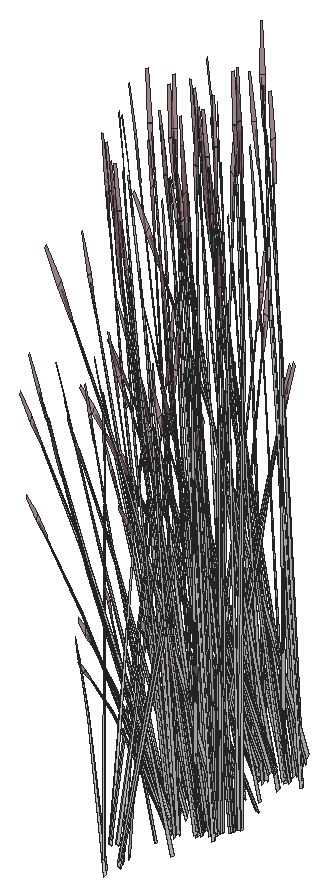
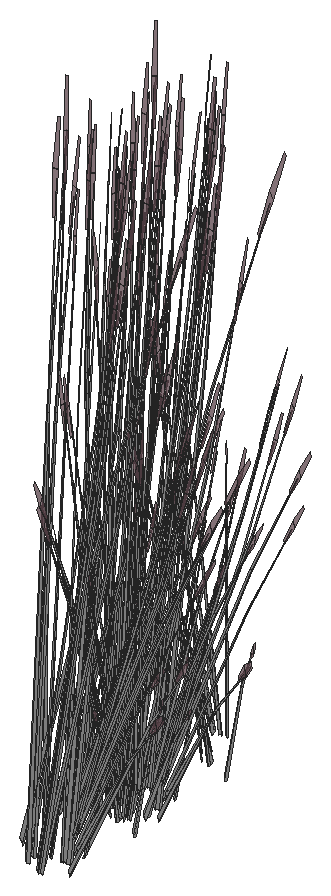
# SketchUp Ruby script. Lengths in inches.
U = 1.inch
M = Sketchup.active_model
def pt(a) = Geom::Point3d.new(a.map { |v| v * U })
def face(e, loops, mat)
  f = e.add_face(loops[0].map { |a| pt(a) })
  loops[1..].each { |l| e.add_face(l.map { |a| pt(a) }).erase! }
  f.material = f.back_material = mat if mat
  f
end
# faces: each face lists its corners as indices into pts; further lists are holes
def faces(e, pts, list, mat = nil) = list.each { |f| face(e, (f[0].is_a?(Array) ? f : [f]).map { |l| l.map { |i| pts[i] } }, mat) }
# xy, xz, yz: faces in a plane at the given z, y or x. An outline is a flat list of corners, or four numbers for a rectangle; further outlines are holes
def ring(l) = l.size == 4 ? [[l[0], l[1]], [l[2], l[1]], [l[2], l[3]], [l[0], l[3]]] : l.each_slice(2).to_a
def flat(e, list, mat, &to3) = list.each { |f| face(e, (f[0].is_a?(Array) ? f : [f]).map { |l| ring(l).map { |u, v| to3.(u, v) } }, mat) }
def xy(e, z, list, mat = nil) = flat(e, list, mat) { |x, y| [x, y, z] }
def xz(e, y, list, mat = nil) = flat(e, list, mat) { |x, z| [x, y, z] }
def yz(e, x, list, mat = nil) = flat(e, list, mat) { |y, z| [x, y, z] }
def lines(e, pts, list) = list.each { |a, b| e.add_line(pt(pts[a]), pt(pts[b])) }
# prism: a flat outline (further loops are holes) pulled along v
def prism(e, loops, v, mat = nil)
  f = face(e, loops, mat); d = Geom::Vector3d.new(v.map { |x| x * U })
  f.pushpull(f.normal.samedirection?(d) ? d.length : -d.length)
end
def box(e, o, s, mat = nil) = prism(e, [[o, [o[0] + s[0], o[1], o[2]], [o[0] + s[0], o[1] + s[1], o[2]], [o[0], o[1] + s[1], o[2]]]], [0, 0, s[2]], mat)
def at(x, y, z, deg = 0) = Geom::Transformation.translation(pt([x, y, z])) * Geom::Transformation.rotation(ORIGIN, Z_AXIS, deg.degrees)
def axes(o, x, y, z) = Geom::Transformation.new([*x, 0, *y, 0, *z, 0, *pt(o).to_a, 1])
def part(name) = M.definitions.add(name)
# library, detail: a bought-in or finely detailed component or shape, given as its bounding box
def library(name, o, s) = part(name).tap { |d| box(d.entities, o, s) }
def detail(e, o, s) = box(e.add_group.entities, o, s)
def put(e, d, t, mat = nil) = e.add_instance(d, t).tap { |i| i.material = mat if mat }
def group(e, t, mat = nil) = e.add_group.tap { |g| g.transformation = t; g.material = mat if mat }.entities
root = M.entities
M.materials.add("LightPink_Translucent").color = [144, 107, 117]
M.materials["LightPink_Translucent"].alpha = 0.75
M.materials.add("[_0053_Ivory_]").color = [200, 200, 200]
c1 = part("blade")
p = [[2.15,0.21,22],[0,0.17,0],[0.09,0.45,0],[2.18,0.31,22],[2.29,0.31,22],[0.38,0.45,0],
  [2.48,0.24,33],[2.49,0.24,33],[2.48,0.22,33]]
faces(c1.entities,p,[[0,1,2,3],[4,5,2,3],[6,3,4,7],[8,0,3,6]])
c2 = part("seeds")
p = [[0.3,-0.1,1.38],[-0.01,-0.03,1.59],[-0.01,-0.03,0.03],[0.14,-0.07,-0.07],[0.29,-0.03,3],[0.15,0.01,3.11]]
faces(c2.entities,p,[[0,1,2,3],[1,0,4,5]],"LightPink_Translucent")
c3 = part("blade with seeds")
put(c3.entities,c1,at(0,0,0))
put(c3.entities,c2,axes([2.4,0.25,30.99],[1.5799,-0.05474,1.17369],[-0.12525,1.92788,0.29478],[-0.07173,-0.02425,1.56792]))
put(root,c3,axes([629.08,314.01,255.53],[0.25192,-0.01424,1.71376],[-0.16712,0.61729,0.13857],[-0.35901,-0.03818,0.73262]),"[_0053_Ivory_]")
put(root,c3,axes([629.08,324.12,255.53],[0.25192,-0.01424,1.71376],[-0.16712,0.61729,0.13857],[-0.35901,-0.03818,0.73262]),"[_0053_Ivory_]")
put(root,c3,axes([629.1875,315.1,255.53],[0.21074,-0.13302,1.71376],[0.17741,0.61464,0.13857],[-0.33083,0.13891,0.73262]),"[_0053_Ivory_]")
put(root,c3,axes([628.53,316.14,254.24],[0.21107,0.05162,1.43002],[0.13604,0.52729,-0.30754],[-0.28671,0.0987,0.61141]),"[_0053_Ivory_]")
put(root,c3,axes([630.4,314.45,255],[0.17264,-0.09097,1.77064],[0.05953,0.63516,0.13857],[-0.37394,0.08428,0.63284]),"[_0053_Ivory_]")
put(root,c3,axes([629.83,313.4375,256.63],[-0.60713,-0.01514,-0.71045],[0.04078,-0.63759,0.08574],[-0.25721,-0.06729,1.00501]),"[_0053_Ivory_]")
put(root,c3,axes([629.83,323.54,256.63],[-0.60713,-0.01514,-0.71045],[0.04078,-0.63759,0.08574],[-0.25721,-0.06729,1.00501]),"[_0053_Ivory_]")
put(root,c3,axes([629.35,313.59,254.24],[0.11858,0.17508,1.43002],[-0.27325,0.4759,-0.30754],[-0.28057,-0.11375,0.61141]),"[_0053_Ivory_]")
put(root,c3,axes([629.35,323.7,254.24],[0.11858,0.17508,1.43002],[-0.27325,0.4759,-0.30754],[-0.28057,-0.11375,0.61141]),"[_0053_Ivory_]")
put(root,c3,axes([628.86,314.54,256.18],[-0.50475,-0.17543,-0.35414],[0.14722,-0.5118,0.4572],[-0.20322,0.04693,0.87481]),"[_0053_Ivory_]")
put(root,c3,axes([628.86,324.65,256.18],[-0.50475,-0.17543,-0.35414],[0.14722,-0.5118,0.4572],[-0.20322,0.04693,0.87481]),"[_0053_Ivory_]")
put(root,c3,axes([629.56,323.125,255.53],[0.2256,0.10835,1.71376],[-0.46687,0.45453,0.13857],[-0.29098,-0.20505,0.73262]),"[_0053_Ivory_]")
put(root,c3,axes([629.21,314.8,256.33],[-0.16454,0.57202,-0.51099],[-0.56413,-0.19607,-0.3958],[-0.22713,0.05245,0.97773]),"[_0053_Ivory_]")
put(root,c3,axes([629.63,313.56,256.33],[-0.44101,0.41656,-0.51099],[-0.38623,-0.44004,-0.3958],[-0.22407,-0.06338,0.97773]),"[_0053_Ivory_]")
put(root,c3,axes([629.63,323.67,256.33],[-0.44101,0.41656,-0.51099],[-0.38623,-0.44004,-0.3958],[-0.22407,-0.06338,0.97773]),"[_0053_Ivory_]")
put(root,c3,axes([628.92,314.76,253.15],[0.0154,0.09911,1.76342],[-0.31051,0.51756,-0.26939],[-0.22056,-0.02609,0.30037]),"[_0053_Ivory_]")
put(root,c3,axes([628.92,324.87,253.15],[0.0154,0.09911,1.76342],[-0.31051,0.51756,-0.26939],[-0.22056,-0.02609,0.30037]),"[_0053_Ivory_]")
put(root,c3,axes([628.09,317.25,254.42],[0.25312,-0.28501,1.1486],[0.09988,0.45119,0.84392],[-0.18292,0.08079,0.25299]),"[_0053_Ivory_]")
put(root,c3,axes([629.47,313.17,256.18],[-0.34557,-0.39372,-0.35414],[0.39459,-0.37271,0.4572],[-0.20048,-0.05671,0.87481]),"[_0053_Ivory_]")
put(root,c3,axes([629.47,323.28,256.18],[-0.34557,-0.39372,-0.35414],[0.39459,-0.37271,0.4572],[-0.20048,-0.05671,0.87481]),"[_0053_Ivory_]")
put(root,c3,axes([629.96,315.51,255.53],[0.1517,-0.19322,1.71376],[0.38303,0.52154,0.13857],[-0.26271,0.23751,0.73262]),"[_0053_Ivory_]")
put(root,c3,axes([629.04,316.02,256.18],[-0.52868,0.08987,-0.35414],[-0.1396,-0.51376,0.4572],[-0.1515,0.13799,0.87481]),"[_0053_Ivory_]")
put(root,c3,axes([628.76,307.15,253.15],[0.08147,0.06283,1.76342],[0.13814,0.58211,-0.26939],[-0.18056,0.12413,0.30037]),"[_0053_Ivory_]")
put(root,c3,axes([628.76,317.54,253.15],[0.08147,0.06283,1.76342],[0.13814,0.58211,-0.26939],[-0.18056,0.12413,0.30037]),"[_0053_Ivory_]")
put(root,c3,axes([628.64,314.12,254.42],[0.38775,-0.045,1.1486],[-0.24596,0.39648,0.84392],[-0.19161,-0.05948,0.25299]),"[_0053_Ivory_]")
put(root,c3,axes([628.64,324.22,254.42],[0.38775,-0.045,1.1486],[-0.24596,0.39648,0.84392],[-0.19161,-0.05948,0.25299]),"[_0053_Ivory_]")
put(root,c3,axes([629.84,305.6,255.53],[0.11309,-0.21615,1.71376],[0.47441,0.44731,0.13857],[-0.21402,0.27879,0.73262]),"[_0053_Ivory_]")
put(root,c3,axes([629.84,315.99,255.53],[0.11309,-0.21615,1.71376],[0.47441,0.44731,0.13857],[-0.21402,0.27879,0.73262]),"[_0053_Ivory_]")
put(root,c3,axes([629.48,316.08,256.33],[0.15602,0.5742,-0.51099],[-0.59087,0.10045,-0.3958],[-0.16933,0.15423,0.97773]),"[_0053_Ivory_]")
put(root,c3,axes([630.95,315.66,253.71],[-0.63179,-0.1031,-0.62353],[0.13332,-0.63596,-0.16365],[-0.18854,-0.07706,1.37633]),"[_0053_Ivory_]")
put(root,c3,axes([630.95,325.77,253.71],[-0.63179,-0.1031,-0.62353],[0.13332,-0.63596,-0.16365],[-0.18854,-0.07706,1.37633]),"[_0053_Ivory_]")
put(root,c3,axes([630.89,322.79,256.63],[-0.51789,-0.30395,-0.71045],[0.36805,-0.53263,0.08574],[-0.18764,-0.18149,1.00501]),"[_0053_Ivory_]")
put(root,c3,axes([630.65,312.7,256.33],[-0.59932,0.14948,-0.51099],[-0.10484,-0.56611,-0.3958],[-0.16097,-0.16223,0.97773]),"[_0053_Ivory_]")
put(root,c3,axes([630.65,322.81,256.33],[-0.59932,0.14948,-0.51099],[-0.10484,-0.56611,-0.3958],[-0.16097,-0.16223,0.97773]),"[_0053_Ivory_]")
put(root,c3,axes([630.125,316.87,253.67],[-0.56842,-0.31443,-0.49651],[0.33976,-0.56381,0],[-0.12946,-0.07161,1.57504]),"[_0053_Ivory_]")
put(root,c3,axes([630.125,326.97,253.67],[-0.56842,-0.31443,-0.49651],[0.33976,-0.56381,0],[-0.12946,-0.07161,1.57504]),"[_0053_Ivory_]")
put(root,c3,axes([629.875,322.29,253.15],[-0.05883,0.08284,1.76342],[-0.59454,0.17861,-0.26939],[-0.14363,-0.16248,0.30037]),"[_0053_Ivory_]")
put(root,c3,axes([630.47,317.25,254.03],[-0.37973,0.63014,0],[-0.6353,-0.35142,-0.51607],[-0.14469,-0.08004,1.63711]),"[_0053_Ivory_]")
put(root,c3,axes([629.78,307.77,254.24],[0.19166,-0.0992,1.43002],[0.4732,0.29912,-0.30754],[-0.14084,0.25882,0.61141]),"[_0053_Ivory_]")
put(root,c3,axes([629.78,318.16,254.24],[0.19166,-0.0992,1.43002],[0.4732,0.29912,-0.30754],[-0.14084,0.25882,0.61141]),"[_0053_Ivory_]")
put(root,c3,axes([629.51,312.5,253.78],[-0.1752,0.51349,-0.03893],[-0.53924,-0.15795,-0.17649],[-0.08187,-0.08399,0.58215]),"[_0053_Ivory_]")
put(root,c3,axes([629.51,322.61,253.78],[-0.1752,0.51349,-0.03893],[-0.53924,-0.15795,-0.17649],[-0.08187,-0.08399,0.58215]),"[_0053_Ivory_]")
put(root,c3,axes([630.3125,321.96,254.24],[-0.03678,0.20572,1.43002],[-0.53767,0.17221,-0.30754],[-0.12568,-0.26589,0.61141]),"[_0053_Ivory_]")
put(root,c3,axes([630.49,322.49,255.53],[0.13883,0.2019,1.71376],[-0.64153,0.16998,0.13857],[-0.14499,-0.31697,0.73262]),"[_0053_Ivory_]")
put(root,c3,axes([631.67,315.76,254.32],[-0.61322,0.4175,-0.29095],[-0.40778,-0.58992,-0.50002],[-0.1513,-0.05991,1.59708]),"[_0053_Ivory_]")
put(root,c3,axes([630.71,322.39,256.18],[-0.0938,-0.50652,-0.35414],[0.53623,-0.13375,0.4572],[-0.14403,-0.14515,0.87481]),"[_0053_Ivory_]")
put(root,c3,axes([629.22,314.85,254.03],[-0.75945,0,0],[0,-0.70283,-0.51607],[0,-0.16007,1.63711]),"[_0053_Ivory_]")
put(root,c3,axes([629.22,324.95,254.03],[-0.75945,0,0],[0,-0.70283,-0.51607],[0,-0.16007,1.63711]),"[_0053_Ivory_]")
put(root,c3,axes([630.28,316.63,253.68],[-0.14267,-0.54795,-0.30978],[0.56663,-0.1556,0.30978],[-0.11423,-0.06319,1.38974]),"[_0053_Ivory_]")
put(root,c3,axes([630.28,326.74,253.68],[-0.14267,-0.54795,-0.30978],[0.56663,-0.1556,0.30978],[-0.11423,-0.06319,1.38974]),"[_0053_Ivory_]")
put(root,c3,axes([629.97,306.8125,256.18],[-0.41095,0.33109,-0.35414],[-0.38901,-0.37805,0.4572],[-0.05919,0.19208,0.87481]),"[_0053_Ivory_]")
put(root,c3,axes([629.97,317.2,256.18],[-0.41095,0.33109,-0.35414],[-0.38901,-0.37805,0.4572],[-0.05919,0.19208,0.87481]),"[_0053_Ivory_]")
put(root,c3,axes([632.08,316.21,253.71],[-0.40909,0.47266,-0.62353],[-0.50819,-0.4286,-0.16365],[-0.16393,0.11791,1.37633]),"[_0053_Ivory_]")
put(root,c3,axes([629.8,314.66,253.98],[-0.56493,0.5287,0.30756],[-0.56528,-0.52313,-0.36492],[-0.01973,-0.15014,1.64885]),"[_0053_Ivory_]")
put(root,c3,axes([629.8,324.77,253.98],[-0.56493,0.5287,0.30756],[-0.56528,-0.52313,-0.36492],[-0.01973,-0.15014,1.64885]),"[_0053_Ivory_]")
put(root,c3,axes([632.13,316.12,254.98],[0.52485,0.25358,1.51261],[-0.51417,0.54629,0.59816],[-0.23031,-0.32378,1.26806]),"[_0053_Ivory_]")
put(root,c3,axes([632.13,326.23,254.98],[0.52485,0.25358,1.51261],[-0.51417,0.54629,0.59816],[-0.23031,-0.32378,1.26806]),"[_0053_Ivory_]")
put(root,c3,axes([630.125,321.63,254.42],[0.31682,0.21887,1.1486],[-0.4614,0.13157,0.84392],[-0.09872,-0.16821,0.25299]),"[_0053_Ivory_]")
put(root,c3,axes([632.36,315.95,254.12],[-0.59306,-0.50614,-0.25192],[0.49904,-0.56836,0.5513],[-0.1597,0.05921,1.68216]),"[_0053_Ivory_]")
put(root,c3,axes([631.28,315.46,253.86],[-0.36485,-0.52782,-0.44739],[0.55265,-0.37168,0.21531],[-0.11807,-0.06531,1.43643]),"[_0053_Ivory_]")
put(root,c3,axes([631.28,325.57,253.86],[-0.36485,-0.52782,-0.44739],[0.55265,-0.37168,0.21531],[-0.11807,-0.06531,1.43643]),"[_0053_Ivory_]")
put(root,c3,axes([630.25,306.46,256.99],[-0.0158,0.58168,-0.7886],[-0.66548,-0.03907,0.09517],[-0.07023,0.24643,1.11556]),"[_0053_Ivory_]")
put(root,c3,axes([630.25,316.85,256.99],[-0.0158,0.58168,-0.7886],[-0.66548,-0.03907,0.09517],[-0.07023,0.24643,1.11556]),"[_0053_Ivory_]")
put(root,c3,axes([630.24,308.1,254.42],[-0.01572,-0.37392,1.1486],[0.39276,0.26669,0.84392],[-0.07724,0.17822,0.25299]),"[_0053_Ivory_]")
put(root,c3,axes([630.24,318.49,254.42],[-0.01572,-0.37392,1.1486],[0.39276,0.26669,0.84392],[-0.07724,0.17822,0.25299]),"[_0053_Ivory_]")
put(root,c3,axes([632.06,315.84,253.86],[-0.65953,0.03882,-0.44739],[-0.05964,-0.64439,0.21531],[-0.11807,0.06531,1.43643]),"[_0053_Ivory_]")
put(root,c3,axes([630.8,316.92,254.13],[0.56842,0.31443,0.49651],[-0.33976,0.56381,0],[-0.12946,-0.07161,1.57504]),"[_0053_Ivory_]")
put(root,c3,axes([630.03,307.28,255.02],[0.01334,-0.32463,1.54345],[0.60018,0.17147,0.21329],[-0.052,0.34598,0.72882]),"[_0053_Ivory_]")
put(root,c3,axes([630.03,317.67,255.02],[0.01334,-0.32463,1.54345],[0.60018,0.17147,0.21329],[-0.052,0.34598,0.72882]),"[_0053_Ivory_]")
put(root,c3,axes([631.33,315.76,254.09],[0.16098,-0.74515,-0.23429],[0.76326,0.12989,0.51271],[-0.13337,-0.1029,1.5644]),"[_0053_Ivory_]")
put(root,c3,axes([631.33,325.87,254.09],[0.16098,-0.74515,-0.23429],[0.76326,0.12989,0.51271],[-0.13337,-0.1029,1.5644]),"[_0053_Ivory_]")
put(root,c3,axes([631.61,315.94,254.27],[-0.11717,0.56122,0.1448],[-0.57245,-0.09742,-0.41347],[-0.10418,-0.05763,1.26744]),"[_0053_Ivory_]")
put(root,c3,axes([632.75,317.5,253.67],[-0.56842,0.31443,-0.49651],[-0.33976,-0.56381,0],[-0.12946,0.07161,1.57504]),"[_0053_Ivory_]")
put(root,c3,axes([629.39,314.37,253.67],[0,-0.62885,-0.49651],[0.67951,0,0],[0,-0.14322,1.57504]),"[_0053_Ivory_]")
put(root,c3,axes([629.39,324.48,253.67],[0,-0.62885,-0.49651],[0.67951,0,0],[0,-0.14322,1.57504]),"[_0053_Ivory_]")
put(root,c3,axes([629.68,314.95,254.13],[0,0.62885,0.49651],[-0.67951,0,0],[0,-0.14322,1.57504]),"[_0053_Ivory_]")
put(root,c3,axes([629.68,325.06,254.13],[0,0.62885,0.49651],[-0.67951,0,0],[0,-0.14322,1.57504]),"[_0053_Ivory_]")
put(root,c3,axes([632.79,317.33,253.85],[-0.37499,-0.63235,-0.05142],[0.6353,-0.35142,0.51607],[-0.15655,0.0602,1.6363]),"[_0053_Ivory_]")
put(root,c3,axes([630.38,306.66,256.66],[0.43478,0.42253,-0.5672],[-0.45929,0.37004,-0.43934],[-0.06615,0.21468,1.08528]),"[_0053_Ivory_]")
put(root,c3,axes([630.38,317.05,256.66],[0.43478,0.42253,-0.5672],[-0.45929,0.37004,-0.43934],[-0.06615,0.21468,1.08528]),"[_0053_Ivory_]")
put(root,c3,axes([632.62,317.25,253.68],[-0.56663,-0.1556,-0.30978],[0.14267,-0.54795,0.30978],[-0.11423,0.06319,1.38974]),"[_0053_Ivory_]")
put(root,c3,axes([631.16,315.1,254.32],[-0.68399,-0.30005,-0.29095],[0.32934,-0.63331,-0.50002],[-0.0215,-0.15549,1.59708]),"[_0053_Ivory_]")
put(root,c3,axes([631.16,325.2,254.32],[-0.68399,-0.30005,-0.29095],[0.32934,-0.63331,-0.50002],[-0.0215,-0.15549,1.59708]),"[_0053_Ivory_]")
put(root,c3,axes([632.94,314.91,254.5],[-0.01659,-0.59209,1.41272],[0.75089,0.15348,0.59816],[-0.1776,0.32398,1.3335]),"[_0053_Ivory_]")
put(root,c3,axes([629.91,307.29,254.48],[0.55175,-0.11136,0.06507],[0.12684,0.44864,-0.86304],[-0.03498,0.22711,0.7736]),"[_0053_Ivory_]")
put(root,c3,axes([629.91,317.68,254.48],[0.55175,-0.11136,0.06507],[0.12684,0.44864,-0.86304],[-0.03498,0.22711,0.7736]),"[_0053_Ivory_]")
put(root,c3,axes([632.52,315.67,254.32],[0.07077,0.71755,-0.29095],[-0.73712,0.04339,-0.50002],[-0.1298,0.09558,1.59708]),"[_0053_Ivory_]")
put(root,c3,axes([630.86,324.57,253.75],[-0.24943,-0.64486,-0.69835],[0.71849,-0.23224,-0.18329],[-0.02757,-0.21836,1.54149]),"[_0053_Ivory_]")
put(root,c3,axes([631.98,322.54,256.33],[-0.59704,-0.15764,-0.51099],[0.20464,-0.54049,-0.3958],[-0.05475,-0.21761,0.97773]),"[_0053_Ivory_]")
put(root,c3,axes([630.88,306.05,255.53],[-0.01487,-0.24136,1.71376],[0.64429,0.16012,0.13857],[-0.03985,0.34396,0.73262]),"[_0053_Ivory_]")
put(root,c3,axes([630.88,316.44,255.53],[-0.01487,-0.24136,1.71376],[0.64429,0.16012,0.13857],[-0.03985,0.34396,0.73262]),"[_0053_Ivory_]")
put(root,c3,axes([629.68,314.38,253.68],[0.42396,-0.39235,-0.30978],[0.42396,0.39235,0.30978],[0,-0.12637,1.38974]),"[_0053_Ivory_]")
put(root,c3,axes([629.68,324.49,253.68],[0.42396,-0.39235,-0.30978],[0.42396,0.39235,0.30978],[0,-0.12637,1.38974]),"[_0053_Ivory_]")
put(root,c3,axes([631.59,311.85,253.78],[-0.4197,0.36076,-0.03893],[-0.38456,-0.39511,-0.17649],[-0.02707,-0.11196,0.58215]),"[_0053_Ivory_]")
put(root,c3,axes([631.59,321.95,253.78],[-0.4197,0.36076,-0.03893],[-0.38456,-0.39511,-0.17649],[-0.02707,-0.11196,0.58215]),"[_0053_Ivory_]")
put(root,c3,axes([631.42,315.4,254.01],[0.76764,0.13249,0.45755],[-0.15622,0.74829,0.17955],[-0.11218,-0.07226,1.58856]),"[_0053_Ivory_]")
put(root,c3,axes([631.42,325.51,254.01],[0.76764,0.13249,0.45755],[-0.15622,0.74829,0.17955],[-0.11218,-0.07226,1.58856]),"[_0053_Ivory_]")
put(root,c3,axes([631.22,315.27,254.37],[-0.29468,0.56664,0.44739],[-0.61229,-0.27271,-0.21531],[0,-0.13062,1.43643]),"[_0053_Ivory_]")
put(root,c3,axes([631.22,325.375,254.37],[-0.29468,0.56664,0.44739],[-0.61229,-0.27271,-0.21531],[0,-0.13062,1.43643]),"[_0053_Ivory_]")
put(root,c3,axes([632.2,322.65,256.63],[-0.28988,-0.51132,-0.71045],[0.59671,-0.28496,0.08574],[-0.06778,-0.24706,1.00501]),"[_0053_Ivory_]")
put(root,c3,axes([631.01,316.6,254.13],[0.65264,-0.16691,0.17642],[0.16115,0.62115,0.35086],[-0.05821,-0.0905,1.60407]),"[_0053_Ivory_]")
put(root,c3,axes([631.01,326.71,254.13],[0.65264,-0.16691,0.17642],[0.16115,0.62115,0.35086],[-0.05821,-0.0905,1.60407]),"[_0053_Ivory_]")
put(root,c3,axes([631.85,316.7,253.85],[-0.61229,-0.28233,0],[0.29468,-0.58663,0],[0,0,1.62707]),"[_0053_Ivory_]")
put(root,c3,axes([633.27,317.41,254.03],[0.37973,0.63014,0],[-0.6353,0.35142,-0.51607],[-0.14469,0.08004,1.63711]),"[_0053_Ivory_]")
put(root,c3,axes([632.95,316.63,254.13],[0.17545,-0.62497,0.17642],[0.64204,0.17686,0.35086],[-0.11091,0.00304,1.60407]),"[_0053_Ivory_]")
put(root,c3,axes([632.66,315.8,254.27],[0.44871,0.37783,0.1448],[-0.37428,0.42627,-0.41347],[-0.10418,0.05763,1.26744]),"[_0053_Ivory_]")
put(root,c3,axes([632.5,315.34,253.95],[-0.56493,-0.54126,-0.06131],[0.56528,-0.54159,0],[-0.01973,-0.0189,1.75571]),"[_0053_Ivory_]")
put(root,c3,axes([632.5,325.44,253.95],[-0.56493,-0.54126,-0.06131],[0.56528,-0.54159,0],[-0.01973,-0.0189,1.75571]),"[_0053_Ivory_]")
put(root,c3,axes([632.65,315.53,254.37],[0.65953,-0.03882,0.44739],[0.05964,0.64439,-0.21531],[-0.11807,0.06531,1.43643]),"[_0053_Ivory_]")
put(root,c3,axes([632.81,317.01,253.98],[0.76036,0.2044,0.30756],[-0.19023,0.7306,-0.36492],[-0.12585,0.09144,1.64885]),"[_0053_Ivory_]")
put(root,c3,axes([631.7,321.51,253.15],[-0.10187,0.02266,1.76342],[-0.56336,-0.25503,-0.26939],[0.00945,-0.21273,0.30037]),"[_0053_Ivory_]")
put(root,c3,axes([633.13,316.97,254.13],[0.56842,-0.31443,0.49651],[0.33976,0.56381,0],[-0.12946,0.07161,1.57504]),"[_0053_Ivory_]")
put(root,c3,axes([632.25,322.21,256.18],[0.1831,-0.48359,-0.35414],[0.53419,0.14105,0.4572],[-0.04898,-0.1947,0.87481]),"[_0053_Ivory_]")
put(root,c3,axes([631.36,314.72,254.01],[0.26406,0.70318,0.45755],[-0.7545,0.24452,0.17955],[0.00922,-0.12921,1.58856]),"[_0053_Ivory_]")
put(root,c3,axes([631.36,324.82,254.01],[0.26406,0.70318,0.45755],[-0.7545,0.24452,0.17955],[0.00922,-0.12921,1.58856]),"[_0053_Ivory_]")
